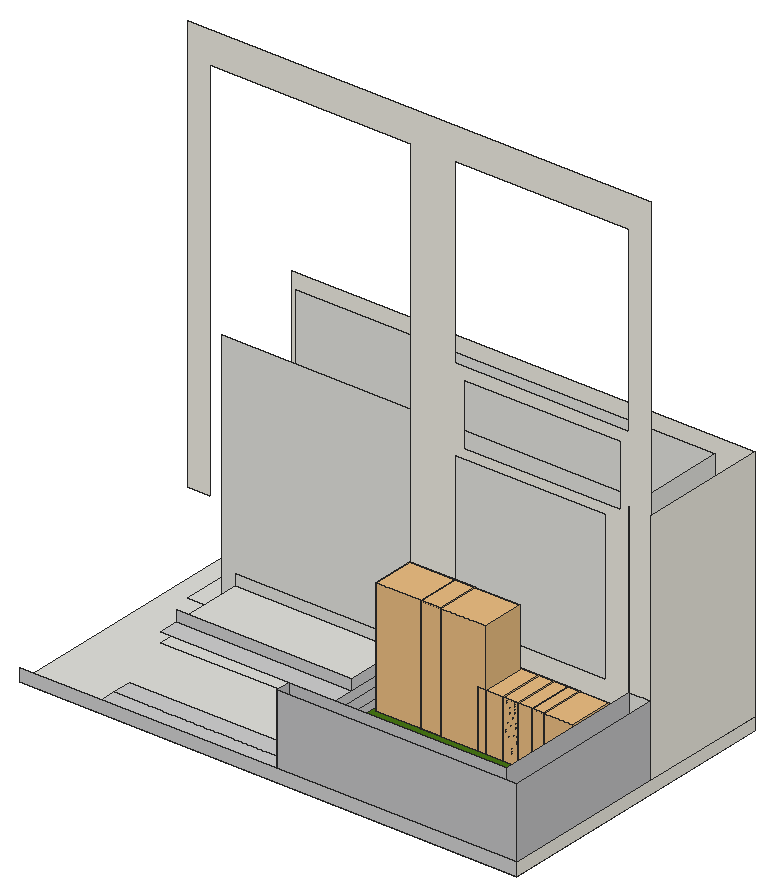
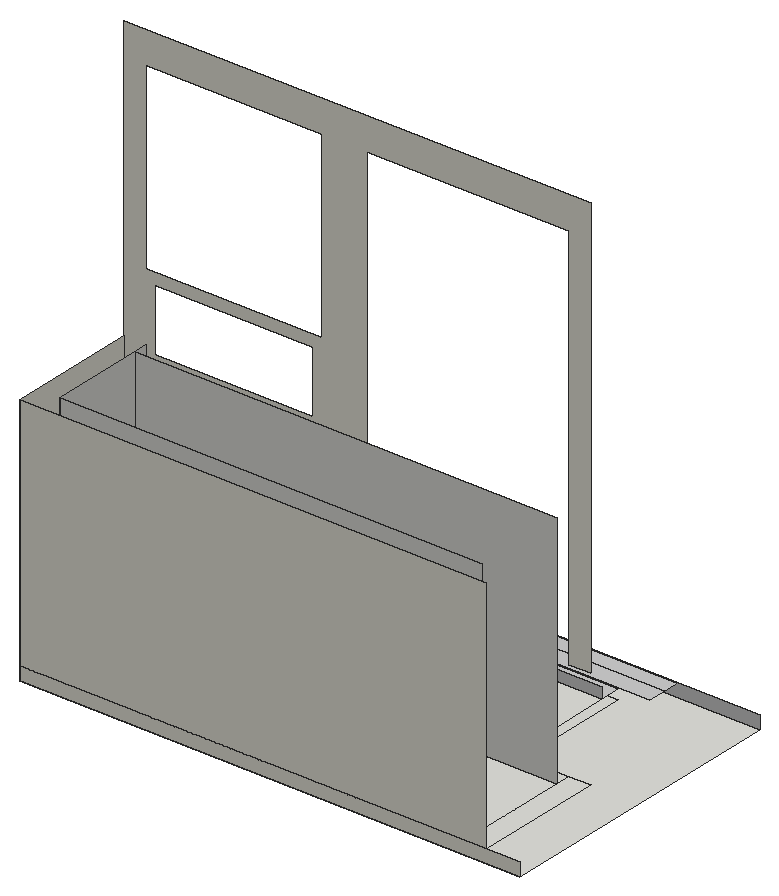
# SketchUp Ruby script. Lengths in inches.
U = 1.inch
M = Sketchup.active_model
def pt(a) = Geom::Point3d.new(a.map { |v| v * U })
def face(e, loops, mat)
  f = e.add_face(loops[0].map { |a| pt(a) })
  loops[1..].each { |l| e.add_face(l.map { |a| pt(a) }).erase! }
  f.material = f.back_material = mat if mat
  f
end
# faces: each face lists its corners as indices into pts; further lists are holes
def faces(e, pts, list, mat = nil) = list.each { |f| face(e, (f[0].is_a?(Array) ? f : [f]).map { |l| l.map { |i| pts[i] } }, mat) }
# xy, xz, yz: faces in a plane at the given z, y or x. An outline is a flat list of corners, or four numbers for a rectangle; further outlines are holes
def ring(l) = l.size == 4 ? [[l[0], l[1]], [l[2], l[1]], [l[2], l[3]], [l[0], l[3]]] : l.each_slice(2).to_a
def flat(e, list, mat, &to3) = list.each { |f| face(e, (f[0].is_a?(Array) ? f : [f]).map { |l| ring(l).map { |u, v| to3.(u, v) } }, mat) }
def xy(e, z, list, mat = nil) = flat(e, list, mat) { |x, y| [x, y, z] }
def xz(e, y, list, mat = nil) = flat(e, list, mat) { |x, z| [x, y, z] }
def yz(e, x, list, mat = nil) = flat(e, list, mat) { |y, z| [x, y, z] }
def lines(e, pts, list) = list.each { |a, b| e.add_line(pt(pts[a]), pt(pts[b])) }
# prism: a flat outline (further loops are holes) pulled along v
def prism(e, loops, v, mat = nil)
  f = face(e, loops, mat); d = Geom::Vector3d.new(v.map { |x| x * U })
  f.pushpull(f.normal.samedirection?(d) ? d.length : -d.length)
end
def box(e, o, s, mat = nil) = prism(e, [[o, [o[0] + s[0], o[1], o[2]], [o[0] + s[0], o[1] + s[1], o[2]], [o[0], o[1] + s[1], o[2]]]], [0, 0, s[2]], mat)
def at(x, y, z, deg = 0) = Geom::Transformation.translation(pt([x, y, z])) * Geom::Transformation.rotation(ORIGIN, Z_AXIS, deg.degrees)
def axes(o, x, y, z) = Geom::Transformation.new([*x, 0, *y, 0, *z, 0, *pt(o).to_a, 1])
def part(name) = M.definitions.add(name)
# library, detail: a bought-in or finely detailed component or shape, given as its bounding box
def library(name, o, s) = part(name).tap { |d| box(d.entities, o, s) }
def detail(e, o, s) = box(e.add_group.entities, o, s)
def put(e, d, t, mat = nil) = e.add_instance(d, t).tap { |i| i.material = mat if mat }
def group(e, t, mat = nil) = e.add_group.tap { |g| g.transformation = t; g.material = mat if mat }.entities
root = M.entities
M.materials.add("[Carrera Marble]").color = [207, 207, 207]
M.materials.add("[Fencing Metal Straight]").color = [194, 195, 196]
M.materials.add("[Tile Limestone Large]").color = [237, 234, 224]
M.materials.add("[Vegetation Honey Locust]").color = [71, 119, 20]
c1 = library("Small+Bush+Planter",[-31.86,3.96,0],[62.63,58.8,106.375])
c2 = library("chau cay",[-24.34,-109.24,0],[56.46,62.58,79.69])
xy(root,0,[[0,0,689.3,413.49]])
xy(root,17.625,[[356.09,0,356.09,21.02,659.08,21.02,659.08,233.86,689.3,233.86,689.3,0],[46.1875,233.86,46.1875,413.49,689.3,413.49,689.3,233.86,659.08,233.86,659.08,383.27,76.4,383.27,76.4,233.86],[76.4,233.86,659.08,254.16],[76.4,254.16,659.08,383.27]])
xy(root,17.625,[[113.3,0,356.09,21.02],[113.3,21.02,355.29,47.98]],"[Carrera Marble]")
xy(root,17.625,[[355.29,21.02,659.08,233.86]],"[Vegetation Honey Locust]")
xy(root,42.68,[[111.93,103.86,355.29,233.86]])
xy(root,56.07,[[111.93,131.48,355.29,233.86]])
xy(root,56.07,[[111.93,103.86,355.29,131.48]],"[Carrera Marble]")
xz(root,0,[[0,0,689.3,17.625]],"[Carrera Marble]")
xz(root,0,[[356.09,17.625,689.3,115.1875]],"[Fencing Metal Straight]")
xz(root,21.02,[[356.09,17.625,659.08,115.1875]],"[Fencing Metal Straight]")
xz(root,131.48,[[111.93,56.07,355.29,70.61]],"[Carrera Marble]")
xz(root,233.86,[[659.08,17.625,689.3,115.1875],[111.93,56.07,355.29,70.61]])
xz(root,233.86,[[[355.29,17.625,659.08,17.625,659.08,115.1875,689.3,115.1875,689.3,737,46.1875,737,46.1875,155.84,76.4,155.84,76.4,692.2,355.29,692.2],[416.36,120.45,416.36,692.2,659.08,692.2,659.08,440.5625,416.36,440.5625,416.36,326.11,627.05,326.11,627.05,120.45],[428.87,338.4,647.75,424.46]]],"[Tile Limestone Large]")
xz(root,254.16,[[76.4,17.625,659.08,346.625]])
xz(root,383.27,[[76.4,17.625,659.08,346.625]])
xz(root,413.49,[[0,0,689.3,17.625],[46.1875,17.625,689.3,346.625]],"[Tile Limestone Large]")
yz(root,355.29,[[47.98,17.625,233.86,28.22],[71.98,28.22,233.86,42.68],[103.86,42.68,233.86,56.07],[131.48,56.07,233.86,70.61]],"[Carrera Marble]")
yz(root,356.09,[[0,17.625,21.02,115.1875]],"[Fencing Metal Straight]")
yz(root,659.08,[[233.86,17.625,254.16,346.625],[254.16,17.625,383.27,346.625]])
yz(root,659.08,[[21.02,17.625,233.86,115.1875]],"[Fencing Metal Straight]")
yz(root,689.3,[[0,17.625,233.86,115.1875]],"[Fencing Metal Straight]")
yz(root,689.3,[[0,0,413.49,17.625],[233.86,17.625,413.49,346.625]],"[Tile Limestone Large]")
put(root,c1,axes([406.83,162.55,17.625],[1.44,0,0],[0,1,0],[0,0,1.5]))
put(root,c1,axes([469.65,162.55,17.625],[1.44,0,0],[0,1,0],[0,0,1.5]))
put(root,c2,at(527.37,274.7,17.625))
put(root,c2,at(562.99,274.7,17.625))
put(root,c2,at(603.12,274.7,17.625))
